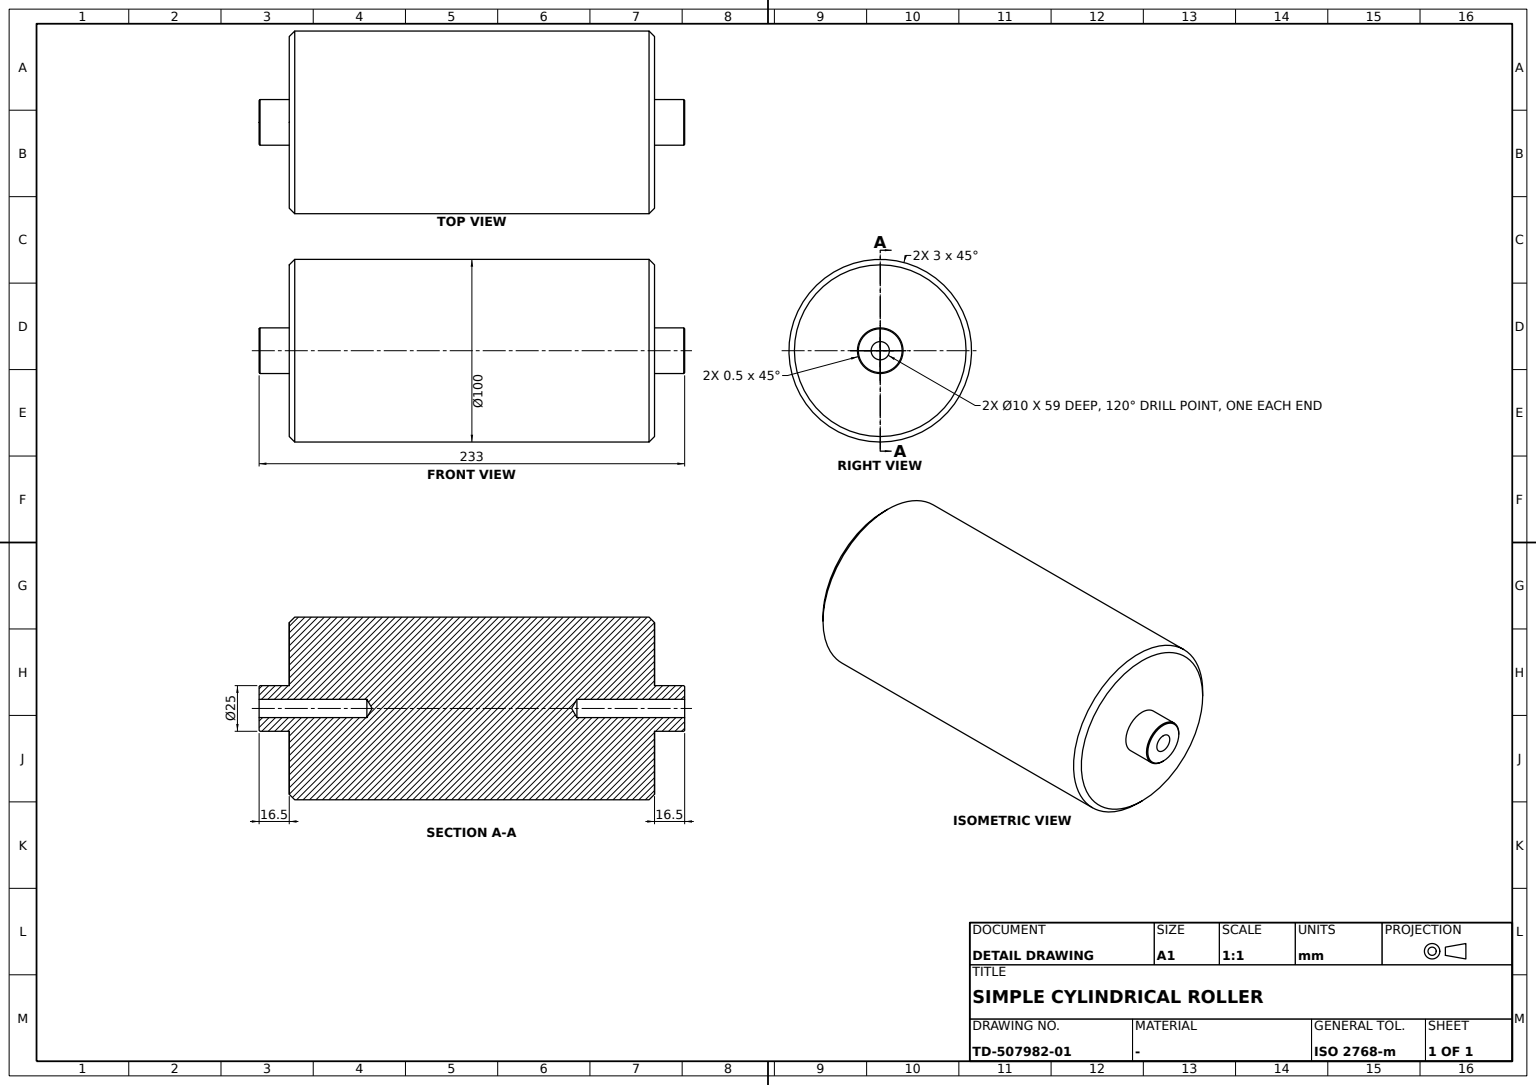
ISO-10303-21;
HEADER;
FILE_DESCRIPTION((''),'2;1');
FILE_NAME('','',(''),(''),'','','');
FILE_SCHEMA(('AUTOMOTIVE_DESIGN'));
ENDSEC;
DATA;
#1=APPLICATION_CONTEXT('');
#2=PRODUCT_CONTEXT('',#1,'mechanical');
#3=PRODUCT('','','',(#2));
#4=PRODUCT_DEFINITION_FORMATION('','',#3);
#5=PRODUCT_DEFINITION_CONTEXT('',#1,'design');
#6=PRODUCT_DEFINITION('','',#4,#5);
#7=PRODUCT_DEFINITION_SHAPE('','',#6);
#8=(LENGTH_UNIT()NAMED_UNIT(*)SI_UNIT(.MILLI.,.METRE.));
#9=(NAMED_UNIT(*)PLANE_ANGLE_UNIT()SI_UNIT($,.RADIAN.));
#10=(NAMED_UNIT(*)SI_UNIT($,.STERADIAN.)SOLID_ANGLE_UNIT());
#11=UNCERTAINTY_MEASURE_WITH_UNIT(LENGTH_MEASURE(0.005),#8,'distance_accuracy_value','');
#12=(GEOMETRIC_REPRESENTATION_CONTEXT(3)GLOBAL_UNCERTAINTY_ASSIGNED_CONTEXT((#11))GLOBAL_UNIT_ASSIGNED_CONTEXT((#8,#9,#10))REPRESENTATION_CONTEXT('',''));
#13=CARTESIAN_POINT('',(0.,116.5,5.));
#14=VERTEX_POINT('',#13);
#15=CARTESIAN_POINT('',(0.,116.5,0.));
#16=DIRECTION('',(0.,1.,0.));
#17=DIRECTION('',(0.,0.,1.));
#18=AXIS2_PLACEMENT_3D('',#15,#16,#17);
#19=CIRCLE('',#18,5.);
#20=EDGE_CURVE('',#14,#14,#19,.T.);
#21=ORIENTED_EDGE('',*,*,#20,.T.);
#22=EDGE_LOOP('',(#21));
#23=FACE_BOUND('',#22,.T.);
#24=CARTESIAN_POINT('',(0.,57.5,5.));
#25=VERTEX_POINT('',#24);
#26=CARTESIAN_POINT('',(0.,57.5,0.));
#27=AXIS2_PLACEMENT_3D('',#26,#16,#17);
#28=CIRCLE('',#27,5.);
#29=EDGE_CURVE('',#25,#25,#28,.F.);
#30=ORIENTED_EDGE('',*,*,#29,.T.);
#31=EDGE_LOOP('',(#30));
#32=FACE_BOUND('',#31,.T.);
#33=CARTESIAN_POINT('',(0.,116.4,0.));
#34=DIRECTION('',(0.,-1.,0.));
#35=DIRECTION('',(1.,0.,0.));
#36=AXIS2_PLACEMENT_3D('',#33,#34,#35);
#37=CYLINDRICAL_SURFACE('',#36,5.);
#38=ADVANCED_FACE('',(#23,#32),#37,.F.);
#39=CARTESIAN_POINT('',(0.,-116.5,5.));
#40=VERTEX_POINT('',#39);
#41=CARTESIAN_POINT('',(0.,-116.5,0.));
#42=AXIS2_PLACEMENT_3D('',#41,#16,#17);
#43=CIRCLE('',#42,5.);
#44=EDGE_CURVE('',#40,#40,#43,.T.);
#45=ORIENTED_EDGE('',*,*,#44,.F.);
#46=EDGE_LOOP('',(#45));
#47=FACE_BOUND('',#46,.T.);
#48=CARTESIAN_POINT('',(0.,-57.5,-5.));
#49=VERTEX_POINT('',#48);
#50=CARTESIAN_POINT('',(0.,-57.5,0.));
#51=DIRECTION('',(0.,0.,-1.));
#52=AXIS2_PLACEMENT_3D('',#50,#34,#51);
#53=CIRCLE('',#52,5.);
#54=EDGE_CURVE('',#49,#49,#53,.F.);
#55=ORIENTED_EDGE('',*,*,#54,.T.);
#56=EDGE_LOOP('',(#55));
#57=FACE_BOUND('',#56,.T.);
#58=ADVANCED_FACE('',(#47,#57),#37,.F.);
#59=CARTESIAN_POINT('',(0.,-54.613249,0.));
#60=VERTEX_POINT('',#59);
#61=VERTEX_LOOP('',#60);
#62=FACE_BOUND('',#61,.T.);
#63=ORIENTED_EDGE('',*,*,#54,.F.);
#64=EDGE_LOOP('',(#63));
#65=FACE_BOUND('',#64,.T.);
#66=AXIS2_PLACEMENT_3D('',#59,#34,#35);
#67=CONICAL_SURFACE('',#66,0.,1.047197551);
#68=ADVANCED_FACE('',(#62,#65),#67,.F.);
#69=CARTESIAN_POINT('',(0.,-100.,47.));
#70=VERTEX_POINT('',#69);
#71=CARTESIAN_POINT('',(0.,-100.,0.));
#72=AXIS2_PLACEMENT_3D('',#71,#16,#17);
#73=CIRCLE('',#72,47.);
#74=EDGE_CURVE('',#70,#70,#73,.T.);
#75=ORIENTED_EDGE('',*,*,#74,.F.);
#76=EDGE_LOOP('',(#75));
#77=FACE_BOUND('',#76,.T.);
#78=CARTESIAN_POINT('',(0.,-100.,12.5));
#79=VERTEX_POINT('',#78);
#80=CIRCLE('',#72,12.5);
#81=EDGE_CURVE('',#79,#79,#80,.T.);
#82=ORIENTED_EDGE('',*,*,#81,.T.);
#83=EDGE_LOOP('',(#82));
#84=FACE_BOUND('',#83,.T.);
#85=DIRECTION('',(-1.,0.,0.));
#86=AXIS2_PLACEMENT_3D('',#71,#16,#85);
#87=PLANE('',#86);
#88=ADVANCED_FACE('',(#77,#84),#87,.F.);
#89=CARTESIAN_POINT('',(0.,-97.,50.));
#90=VERTEX_POINT('',#89);
#91=CARTESIAN_POINT('',(0.,-97.,0.));
#92=AXIS2_PLACEMENT_3D('',#91,#16,#17);
#93=CIRCLE('',#92,50.);
#94=EDGE_CURVE('',#90,#90,#93,.T.);
#95=ORIENTED_EDGE('',*,*,#94,.F.);
#96=EDGE_LOOP('',(#95));
#97=FACE_BOUND('',#96,.T.);
#98=ORIENTED_EDGE('',*,*,#74,.T.);
#99=EDGE_LOOP('',(#98));
#100=FACE_BOUND('',#99,.T.);
#101=CARTESIAN_POINT('',(0.,-147.,0.));
#102=DIRECTION('',(0.963838288,0.,0.266487815));
#103=AXIS2_PLACEMENT_3D('',#101,#16,#102);
#104=CONICAL_SURFACE('',#103,0.,0.785398163);
#105=ADVANCED_FACE('',(#97,#100),#104,.T.);
#106=CARTESIAN_POINT('',(12.5,116.,0.));
#107=VERTEX_POINT('',#106);
#108=CARTESIAN_POINT('',(0.,116.,0.));
#109=AXIS2_PLACEMENT_3D('',#108,#34,#35);
#110=CIRCLE('',#109,12.5);
#111=EDGE_CURVE('',#107,#107,#110,.F.);
#112=ORIENTED_EDGE('',*,*,#111,.F.);
#113=EDGE_LOOP('',(#112));
#114=FACE_BOUND('',#113,.T.);
#115=CARTESIAN_POINT('',(0.,100.,12.5));
#116=VERTEX_POINT('',#115);
#117=CARTESIAN_POINT('',(0.,100.,0.));
#118=AXIS2_PLACEMENT_3D('',#117,#16,#17);
#119=CIRCLE('',#118,12.5);
#120=EDGE_CURVE('',#116,#116,#119,.T.);
#121=ORIENTED_EDGE('',*,*,#120,.T.);
#122=EDGE_LOOP('',(#121));
#123=FACE_BOUND('',#122,.T.);
#124=CARTESIAN_POINT('',(0.,108.25,0.));
#125=AXIS2_PLACEMENT_3D('',#124,#16,#85);
#126=CYLINDRICAL_SURFACE('',#125,12.5);
#127=ADVANCED_FACE('',(#114,#123),#126,.T.);
#128=ORIENTED_EDGE('',*,*,#29,.F.);
#129=EDGE_LOOP('',(#128));
#130=FACE_BOUND('',#129,.T.);
#131=CARTESIAN_POINT('',(0.,54.613249,0.));
#132=VERTEX_POINT('',#131);
#133=VERTEX_LOOP('',#132);
#134=FACE_BOUND('',#133,.T.);
#135=AXIS2_PLACEMENT_3D('',#131,#16,#35);
#136=CONICAL_SURFACE('',#135,0.,1.047197551);
#137=ADVANCED_FACE('',(#130,#134),#136,.F.);
#138=ORIENTED_EDGE('',*,*,#20,.F.);
#139=EDGE_LOOP('',(#138));
#140=FACE_BOUND('',#139,.T.);
#141=CARTESIAN_POINT('',(0.,116.5,12.));
#142=VERTEX_POINT('',#141);
#143=CIRCLE('',#18,12.);
#144=EDGE_CURVE('',#142,#142,#143,.T.);
#145=ORIENTED_EDGE('',*,*,#144,.T.);
#146=EDGE_LOOP('',(#145));
#147=FACE_BOUND('',#146,.T.);
#148=AXIS2_PLACEMENT_3D('',#15,#16,#85);
#149=PLANE('',#148);
#150=ADVANCED_FACE('',(#140,#147),#149,.T.);
#151=ORIENTED_EDGE('',*,*,#144,.F.);
#152=EDGE_LOOP('',(#151));
#153=FACE_BOUND('',#152,.T.);
#154=ORIENTED_EDGE('',*,*,#111,.T.);
#155=EDGE_LOOP('',(#154));
#156=FACE_BOUND('',#155,.T.);
#157=CARTESIAN_POINT('',(0.,128.5,0.));
#158=DIRECTION('',(-0.860070031,0.,-0.510175991));
#159=AXIS2_PLACEMENT_3D('',#157,#34,#158);
#160=CONICAL_SURFACE('',#159,0.,0.785398163);
#161=ADVANCED_FACE('',(#153,#156),#160,.T.);
#162=ORIENTED_EDGE('',*,*,#81,.F.);
#163=EDGE_LOOP('',(#162));
#164=FACE_BOUND('',#163,.T.);
#165=CARTESIAN_POINT('',(-12.5,-116.,0.));
#166=VERTEX_POINT('',#165);
#167=CARTESIAN_POINT('',(0.,-116.,0.));
#168=AXIS2_PLACEMENT_3D('',#167,#16,#85);
#169=CIRCLE('',#168,12.5);
#170=EDGE_CURVE('',#166,#166,#169,.T.);
#171=ORIENTED_EDGE('',*,*,#170,.T.);
#172=EDGE_LOOP('',(#171));
#173=FACE_BOUND('',#172,.T.);
#174=ADVANCED_FACE('',(#164,#173),#126,.T.);
#175=ORIENTED_EDGE('',*,*,#94,.T.);
#176=EDGE_LOOP('',(#175));
#177=FACE_BOUND('',#176,.T.);
#178=CARTESIAN_POINT('',(0.,97.,-50.));
#179=VERTEX_POINT('',#178);
#180=CARTESIAN_POINT('',(0.,97.,0.));
#181=AXIS2_PLACEMENT_3D('',#180,#34,#51);
#182=CIRCLE('',#181,50.);
#183=EDGE_CURVE('',#179,#179,#182,.F.);
#184=ORIENTED_EDGE('',*,*,#183,.F.);
#185=EDGE_LOOP('',(#184));
#186=FACE_BOUND('',#185,.T.);
#187=CARTESIAN_POINT('',(0.,0.,0.));
#188=AXIS2_PLACEMENT_3D('',#187,#16,#85);
#189=CYLINDRICAL_SURFACE('',#188,50.);
#190=ADVANCED_FACE('',(#177,#186),#189,.T.);
#191=ORIENTED_EDGE('',*,*,#183,.T.);
#192=EDGE_LOOP('',(#191));
#193=FACE_BOUND('',#192,.T.);
#194=CARTESIAN_POINT('',(0.,100.,47.));
#195=VERTEX_POINT('',#194);
#196=CIRCLE('',#118,47.);
#197=EDGE_CURVE('',#195,#195,#196,.T.);
#198=ORIENTED_EDGE('',*,*,#197,.F.);
#199=EDGE_LOOP('',(#198));
#200=FACE_BOUND('',#199,.T.);
#201=CARTESIAN_POINT('',(0.,147.,0.));
#202=DIRECTION('',(-0.890625175,0.,-0.454738163));
#203=AXIS2_PLACEMENT_3D('',#201,#34,#202);
#204=CONICAL_SURFACE('',#203,0.,0.785398163);
#205=ADVANCED_FACE('',(#193,#200),#204,.T.);
#206=CARTESIAN_POINT('',(0.,-116.5,12.));
#207=VERTEX_POINT('',#206);
#208=CIRCLE('',#42,12.);
#209=EDGE_CURVE('',#207,#207,#208,.T.);
#210=ORIENTED_EDGE('',*,*,#209,.T.);
#211=EDGE_LOOP('',(#210));
#212=FACE_BOUND('',#211,.T.);
#213=ORIENTED_EDGE('',*,*,#170,.F.);
#214=EDGE_LOOP('',(#213));
#215=FACE_BOUND('',#214,.T.);
#216=CARTESIAN_POINT('',(0.,-128.5,0.));
#217=DIRECTION('',(0.860070031,0.,0.510175991));
#218=AXIS2_PLACEMENT_3D('',#216,#16,#217);
#219=CONICAL_SURFACE('',#218,0.,0.785398163);
#220=ADVANCED_FACE('',(#212,#215),#219,.T.);
#221=ORIENTED_EDGE('',*,*,#197,.T.);
#222=EDGE_LOOP('',(#221));
#223=FACE_BOUND('',#222,.T.);
#224=ORIENTED_EDGE('',*,*,#120,.F.);
#225=EDGE_LOOP('',(#224));
#226=FACE_BOUND('',#225,.T.);
#227=AXIS2_PLACEMENT_3D('',#117,#16,#85);
#228=PLANE('',#227);
#229=ADVANCED_FACE('',(#223,#226),#228,.T.);
#230=ORIENTED_EDGE('',*,*,#44,.T.);
#231=EDGE_LOOP('',(#230));
#232=FACE_BOUND('',#231,.T.);
#233=ORIENTED_EDGE('',*,*,#209,.F.);
#234=EDGE_LOOP('',(#233));
#235=FACE_BOUND('',#234,.T.);
#236=AXIS2_PLACEMENT_3D('',#41,#16,#85);
#237=PLANE('',#236);
#238=ADVANCED_FACE('',(#232,#235),#237,.F.);
#239=CLOSED_SHELL('',(#38,#58,#68,#88,#105,#127,#137,#150,#161,#174,#190,#205,#220,#229,#238));
#240=MANIFOLD_SOLID_BREP('',#239);
#241=ADVANCED_BREP_SHAPE_REPRESENTATION('',(#240),#12);
#242=SHAPE_DEFINITION_REPRESENTATION(#7,#241);
ENDSEC;
END-ISO-10303-21;
